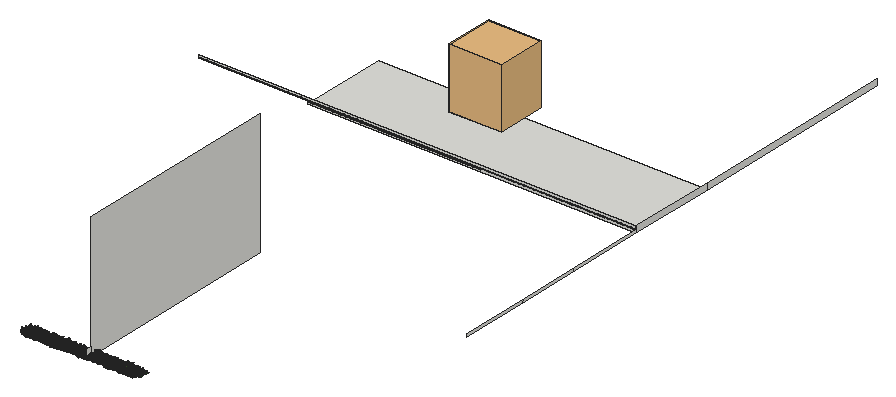
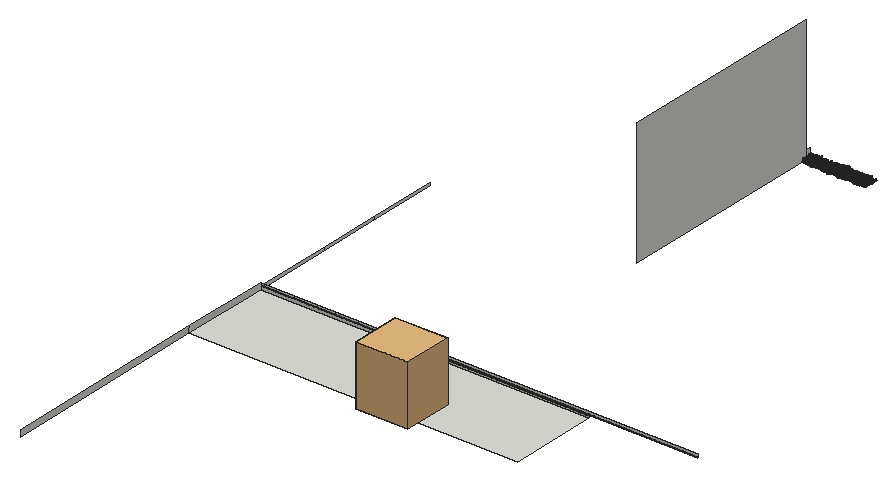
# SketchUp Ruby script. Lengths in inches.
U = 1.inch
M = Sketchup.active_model
def pt(a) = Geom::Point3d.new(a.map { |v| v * U })
def face(e, loops, mat)
  f = e.add_face(loops[0].map { |a| pt(a) })
  loops[1..].each { |l| e.add_face(l.map { |a| pt(a) }).erase! }
  f.material = f.back_material = mat if mat
  f
end
# faces: each face lists its corners as indices into pts; further lists are holes
def faces(e, pts, list, mat = nil) = list.each { |f| face(e, (f[0].is_a?(Array) ? f : [f]).map { |l| l.map { |i| pts[i] } }, mat) }
# xy, xz, yz: faces in a plane at the given z, y or x. An outline is a flat list of corners, or four numbers for a rectangle; further outlines are holes
def ring(l) = l.size == 4 ? [[l[0], l[1]], [l[2], l[1]], [l[2], l[3]], [l[0], l[3]]] : l.each_slice(2).to_a
def flat(e, list, mat, &to3) = list.each { |f| face(e, (f[0].is_a?(Array) ? f : [f]).map { |l| ring(l).map { |u, v| to3.(u, v) } }, mat) }
def xy(e, z, list, mat = nil) = flat(e, list, mat) { |x, y| [x, y, z] }
def xz(e, y, list, mat = nil) = flat(e, list, mat) { |x, z| [x, y, z] }
def yz(e, x, list, mat = nil) = flat(e, list, mat) { |y, z| [x, y, z] }
def lines(e, pts, list) = list.each { |a, b| e.add_line(pt(pts[a]), pt(pts[b])) }
# prism: a flat outline (further loops are holes) pulled along v
def prism(e, loops, v, mat = nil)
  f = face(e, loops, mat); d = Geom::Vector3d.new(v.map { |x| x * U })
  f.pushpull(f.normal.samedirection?(d) ? d.length : -d.length)
end
def box(e, o, s, mat = nil) = prism(e, [[o, [o[0] + s[0], o[1], o[2]], [o[0] + s[0], o[1] + s[1], o[2]], [o[0], o[1] + s[1], o[2]]]], [0, 0, s[2]], mat)
def at(x, y, z, deg = 0) = Geom::Transformation.translation(pt([x, y, z])) * Geom::Transformation.rotation(ORIGIN, Z_AXIS, deg.degrees)
def axes(o, x, y, z) = Geom::Transformation.new([*x, 0, *y, 0, *z, 0, *pt(o).to_a, 1])
def part(name) = M.definitions.add(name)
# library, detail: a bought-in or finely detailed component or shape, given as its bounding box
def library(name, o, s) = part(name).tap { |d| box(d.entities, o, s) }
def detail(e, o, s) = box(e.add_group.entities, o, s)
def put(e, d, t, mat = nil) = e.add_instance(d, t).tap { |i| i.material = mat if mat }
def group(e, t, mat = nil) = e.add_group.tap { |g| g.transformation = t; g.material = mat if mat }.entities
root = M.entities
M.materials.add("Material82").color = [68, 110, 58]
M.materials.add("Material83").color = [48, 90, 38]
M.materials.add("Material84").color = [68, 110, 48]
M.materials.add("Material85").color = [48, 90, 48]
M.materials.add("Material86").color = [58, 110, 58]
M.materials.add("Material87").color = [58, 90, 38]
M.materials.add("Material88").color = [68, 100, 58]
M.materials.add("Material89").color = [48, 100, 38]
c1 = part("grass00")
p = [[-0.6875,0.15,0],[-0.56,0.08,5.52],[-0.04,0.03,2.76],[0.48,-0.02,0],[0.35,-0.02,5.52],[-0.1,-0.14,5.52],
  [-0.12,0.65,8.37],[-0.42,0.65,8.37]]
faces(c1.entities,p,[[0,1,2,3],[3,2,4],[1,5,2],[5,4,2],[1,6,5],[4,5,6],[7,6,1]])
c2 = part("Group16\#1")
put(c2.entities,c1,axes([1.44,-0.61,-0.01],[0.05352,0.12609,0],[-0.10704,0.04543,0.07239],[0.06664,-0.02828,0.11628]),"Material85")
put(c2.entities,c1,axes([0.76,-0.15,-0.01],[0.04676,0.24062,0],[-0.23162,0.04501,0.06642],[0.0652,-0.01267,0.23595]),"Material82")
put(c2.entities,c1,axes([0.79,0.01,-0.01],[-0.00606,0.34651,0],[-0.34381,-0.00602,0.0432],[0.04319,0.00076,0.34386]))
put(c2.entities,c1,axes([1,0.23,-0.01],[-0.07192,0.31144,0],[-0.28722,-0.06632,0.1236],[0.12043,0.02781,0.29478]),"Material84")
put(c2.entities,c1,axes([1.66,0.77,-0.01],[-0.13828,0.29651,0],[-0.21551,-0.1005,0.22471],[0.20365,0.09498,0.23779]),"Material89")
put(c2.entities,c1,axes([0.6875,0.52,-0.01],[-0.18126,0.24051,0],[-0.22746,-0.17142,0.09788],[0.07817,0.05891,0.28481]),"Material84")
put(c2.entities,c1,axes([0.68,0.78,-0.01],[-0.215,0.18688,0],[-0.12385,-0.14248,0.21334],[0.13995,0.16101,0.18878]),"Material82")
put(c2.entities,c1,axes([0.56,1,-0.01],[-0.13756,0.07624,0],[-0.06159,-0.11112,0.0927],[0.04494,0.08108,0.12705]),"Material84")
put(c2.entities,c1,axes([0.2,0.64,-0.01],[-0.23729,0.07254,0],[-0.05711,-0.18681,0.153],[0.04473,0.14632,0.19535]),"Material89")
put(c2.entities,c1,axes([0.0625,0.72,-0.01],[-0.28874,0.02525,0],[-0.02179,-0.24916,0.14647],[0.01276,0.14591,0.25012]),"Material82")
put(c2.entities,c1,axes([-0.08,0.62,-0.01],[-0.34089,-0.04187,0],[0.03255,-0.26504,0.216],[-0.02633,0.21439,0.26703]),"Material89")
put(c2.entities,c1,axes([-0.34,0.98,-0.01],[-0.14314,-0.0493,0],[0.04397,-0.12769,0.06843],[-0.02228,0.0647,0.13505]),"Material89")
put(c2.entities,c1,axes([-0.87,1.45,-0.01],[-0.23488,-0.14114,0],[0.13761,-0.22901,0.06087],[-0.03135,0.05217,0.26717]))
put(c2.entities,c1,axes([-0.72,0.77,-0.01],[-0.14208,-0.13251,0],[0.07209,-0.0773,0.16301],[-0.11118,0.11922,0.1057]),"Material89")
put(c2.entities,c1,axes([-0.62,0.43,-0.01],[-0.14845,-0.21203,0],[0.18654,-0.13061,0.12304],[-0.10079,0.07057,0.22772]),"Material82")
put(c2.entities,c1,axes([-0.68,0.29,-0.01],[-0.13639,-0.32136,0],[0.31723,-0.13464,0.05579],[-0.05136,0.0218,0.34462]),"Material83")
put(c2.entities,c1,axes([-0.64,0.125,-0.01],[-0.0458,-0.23569,0],[0.22124,-0.043,0.08276],[-0.08124,0.01579,0.22538]),"Material86")
put(c2.entities,c1,axes([-1.6,-0.03,-0.01],[0.00576,-0.32897,0],[0.27526,0.00482,0.18018],[-0.18015,-0.00315,0.2753]),"Material84")
put(c2.entities,c1,axes([-1.36,-0.31,-0.01],[0.05718,-0.24765,0],[0.18172,0.04196,0.17267],[-0.16825,-0.03885,0.1865]),"Material89")
put(c2.entities,c1,axes([-1.54,-0.72,-0.01],[0.06537,-0.14017,0],[0.13555,0.06321,0.03939],[-0.0357,-0.01665,0.14956]))
put(c2.entities,c1,axes([-1.19,-0.9,-0.01],[0.09597,-0.12735,0],[0.11214,0.08451,0.07557],[-0.06035,-0.04548,0.14042]),"Material88")
put(c2.entities,c1,axes([-0.47,-0.54,-0.01],[0.11588,-0.10072,0],[0.0618,0.0711,0.12124],[-0.07953,-0.0915,0.0942]))
put(c2.entities,c1,axes([-0.47,-0.84,-0.01],[0.11927,-0.0661,0],[0.06603,0.11913,0.00646],[-0.00313,-0.00565,0.13621]),"Material84")
put(c2.entities,c1,axes([-0.38,-1.24,-0.01],[0.28037,-0.08571,0],[0.0618,0.20215,0.20315],[-0.05939,-0.19428,0.21139]),"Material88")
put(c2.entities,c1,axes([-0.06,-0.66,-0.01],[0.22719,-0.01987,0],[0.01247,0.14255,0.17758],[-0.01547,-0.17691,0.1431]),"Material87")
put(c2.entities,c1,axes([0.11,-0.89,-0.01],[0.14882,0.01828,0],[-0.01058,0.08611,0.12229],[0.01491,-0.12138,0.08676]),"Material85")
put(c2.entities,c1,axes([0.25,-0.72,-0.01],[0.20481,0.07053,0],[-0.06206,0.18022,0.10291],[0.03351,-0.0973,0.1906]),"Material85")
put(c2.entities,c1,axes([0.85,-1.42,-0.01],[0.16481,0.09904,0],[-0.09472,0.15762,0.05616],[0.02893,-0.04814,0.18389]),"Material84")
put(c2.entities,c1,axes([1.01,-1.09,-0.01],[0.21858,0.20385,0],[-0.17495,0.1876,0.15339],[0.10462,-0.11218,0.25652]),"Material89")
put(c2.entities,c1,axes([1.01,-0.71,-0.01],[0.08733,0.12473,0],[-0.06445,0.04512,0.13037],[0.1068,-0.07477,0.07867]),"Material85")
c3 = part("Group15\#1")
put(c3.entities,c2,at(0,0,0))
c4 = part("3darcstudiotree_grass00\#1")
put(c4.entities,c3,at(0,0,0))
c5 = library("Flora+17",[-57.52,158.6,-38.64],[66.99,62.88,77.28])
xy(root,-37.75,[[626.34,932.5,1048.3125,1046.93]])
xz(root,932.5,[[626.34,-37.75,1048.3125,-37.75,1048.3125,-34.17,848.625,-34.17,848.625,-34.6875,626.34,-34.6875],[626.34,-34.6875,848.625,-34.17],[626.34,-34.17,1048.3125,-33.75],[486.07,-33.75,1048.3125,-33.42],[486.07,-33.42,1048.3125,-32.8],
  [486.07,-32.8,1048.3125,-29.74]])
yz(root,782.78,[[381.72,-34.17,387.84,-22.8],[387.84,-34.17,659.09,126.75]])
yz(root,1048.3125,[[660.69,-37.75,750.06,-34.75],[750.06,-37.75,831.37,-34.75],[831.37,-37.75,932.5,-34.17],[932.5,-37.75,1046.93,-37.75,1046.93,-29.74,932.62,-29.74,932.62,-33.625,932.5,-33.625],[1046.93,-37.75,1318.18,-29.74],
  [932.5,-33.625,932.62,-29.74]])
put(root,c4,axes([730.45,381.9375,-34.17],[4.09331,0.01199,0],[-0.0289,1.53398,-0.04293],[-0.00148,0.07869,1.35522]))
put(root,c4,axes([778.3125,381.87,-34.17],[-3.29126,-0.79109,0],[1.80045,-1.16502,-0.03312],[0.11366,-0.07354,1.70984]))
put(root,c4,axes([741.45,381.79,-34.17],[1.86032,1.34861,0],[-2.96544,0.63621,-0.01685],[-0.11323,0.02429,1.93576]))
put(root,c4,axes([736.73,381.58,-34.17],[-4.56188,0.50767,0],[-1.2186,-1.7031,-0.00145],[-0.00214,-0.00299,1.8291]))
put(root,c4,axes([707.26,382.11,-34.17],[-1.58728,-1.19948,0],[3.58979,-0.73882,-0.00435],[0.01908,-0.00393,1.50222]))
put(root,c4,axes([720.02,382,-34.17],[-3.20908,-0.65771,0],[1.52004,-1.1535,-0.02241],[0.0705,-0.0535,1.68548]))
put(root,c4,axes([811.23,381.91,-34.17],[0.845,1.5364,0],[-3.22221,0.27563,-0.00976],[-0.06274,0.00537,1.62508]))
put(root,c4,axes([749.48,382.19,-34.17],[-3.10229,-1.16988,0],[2.93363,-1.20992,-0.00934],[0.03186,-0.01314,1.57129]))
put(root,c4,axes([835.72,382.97,-34.17],[3.21747,0.34612,0],[-1.00705,1.45598,-0.00322],[-0.00588,0.0085,1.99197]))
put(root,c4,axes([807.45,383.26,-34.17],[2.05313,-1.14667,0],[3.04328,0.84748,-0.00946],[0.04471,0.01245,1.61646]))
put(root,c4,axes([710.89,382.88,-34.17],[1.49785,1.29889,0],[-3.32043,0.59552,-0.00419],[-0.02419,0.00434,1.73548]))
put(root,c4,axes([828.28,383.19,-34.17],[-2.06721,-1.47479,0],[2.97534,-0.64864,-0.04183],[0.21369,-0.04658,1.48723]))
put(root,c4,axes([756.44,383.36,-34.17],[3.7963,-0.32727,0],[0.82791,1.49367,-0.02018],[0.02229,0.04022,1.50307]))
put(root,c4,axes([766.5,383.2,-34.17],[3.44974,0.13102,0],[-0.35474,1.45265,-0.03978],[-0.02715,0.11118,1.9745]))
put(root,c4,axes([814.17,383.25,-34.17],[3.55632,0.05998,0],[-0.17821,1.64336,-0.05798],[-0.01271,0.11725,1.60438]))
put(root,c4,axes([838.5,382.91,-34.17],[-3.26011,-0.21751,0],[0.57833,-1.34815,-0.02254],[0.02017,-0.04702,1.39425]))
put(root,c4,axes([773.79,383.16,-34.17],[-2.04014,-1.04561,0],[3.14641,-0.95481,-0.03027],[0.11908,-0.03613,1.47708]))
put(root,c4,axes([750.16,382.96,-34.17],[-4.12072,-0.27119,0],[0.6549,-1.54771,-0.03361],[0.02858,-0.06755,1.54092]))
put(root,c4,axes([707.83,383.13,-34.17],[-3.19208,-0.59663,0],[1.68588,-1.40285,-0.03887],[0.08271,-0.06882,1.46596]))
put(root,c4,axes([717.11,383.21,-34.17],[-3.36658,1.12781,0],[-2.16506,-1.00516,-0.00331],[-0.01262,-0.00586,1.47415]))
put(root,c4,axes([723.95,383.34,-34.17],[-3.68407,-0.02356,0],[0.06081,-1.47897,-0.00434],[0.00034,-0.00838,1.37632]))
put(root,c4,axes([795.54,384.11,-34.17],[3.71353,-0.51552,0],[1.56304,1.75115,-0.03514],[0.05159,0.0578,1.55988]))
put(root,c4,axes([747.36,383.45,-34.17],[0.6827,1.82438,0],[-3.27697,0.19072,-0.00575],[-0.03023,0.00176,1.31904]))
put(root,c4,axes([741.45,383.66,-34.17],[2.40726,1.00896,0],[-2.45133,0.90962,-0.04643],[-0.23456,0.08704,1.7498]))
put(root,c4,axes([734.375,384.03,-34.17],[0.00434,-1.45328,0],[3.77222,0.00175,-0.01884],[0.09694,0.00004,1.45492]))
put(root,c4,axes([817.26,384.18,-34.17],[1.06558,-1.7102,0],[3.88793,0.37676,-0.05295],[0.33853,0.03281,1.97565]))
put(root,c4,axes([763.28,383.8,-34.17],[-4.10821,-0.63147,0],[1.40621,-1.42285,-0.03755],[0.0732,-0.07407,1.55797]))
put(root,c4,axes([779.07,384.18,-34.17],[3.5779,0.22372,0],[-0.65952,1.64048,-0.02805],[-0.02776,0.06904,1.99488]))
put(root,c4,axes([790,384.14,-34.17],[-0.99859,-1.42329,0],[3.17499,-0.34645,-0.0133],[0.07574,-0.00827,1.45899]))
put(root,c4,axes([785.29,383.61,-34.17],[-2.82382,0.83563,0],[-2.68315,-1.4102,-0.02868],[-0.0714,-0.03753,1.39]))
put(root,c4,axes([824.1875,383.98,-34.17],[-4.01729,-0.17274,0],[0.40562,-1.46709,-0.05296],[0.03317,-0.11998,1.62079]))
put(root,c4,axes([729.49,383.9,-34.17],[-4.10797,-0.04724,0],[0.09871,-1.33508,-0.0193],[0.00442,-0.0598,1.99558]))
put(root,c4,axes([801.06,384.04,-34.17],[-1.96777,1.0795,0],[-3.29786,-0.93497,-0.0015],[-0.00541,-0.00153,1.35234]))
put(root,c4,axes([768.48,385.02,-34.17],[0.94515,-1.66762,0],[4.07339,0.35906,-0.0396],[0.18346,0.01617,1.48525]))
put(root,c4,axes([818.375,385.11,-34.17],[3.84561,-0.02617,0],[0.07345,1.67847,-0.0287],[0.00308,0.07036,1.98369]))
put(root,c4,axes([794.87,385.32,-34.17],[1.96372,-1.5045,0],[4.10696,0.83372,-0.06088],[0.26019,0.05282,1.6642]))
put(root,c4,axes([807.73,385.28,-34.17],[3.54187,-0.26159,0],[0.80325,1.69151,-0.05648],[0.04449,0.09368,1.39957]))
put(root,c4,axes([778,385.49,-34.17],[0.99321,-1.58581,0],[3.96504,0.38623,-0.04714],[0.20087,0.01957,1.34372]))
put(root,c4,axes([763.58,385.62,-34.17],[-0.45128,-1.33361,0],[4.22591,-0.22241,-0.03174],[0.17504,-0.00921,1.77768]))
put(root,c4,axes([745.49,385.82,-34.17],[3.22644,-0.51746,0],[1.32565,1.28555,-0.02601],[0.05462,0.05297,1.4702]))
put(root,c4,axes([725.2,385.76,-34.17],[3.6798,1.00569,0],[-2.52504,1.43694,-0.01195],[-0.02817,0.01603,1.37528]))
put(root,c4,axes([789.81,385.57,-34.17],[1.82247,1.66574,0],[-4.14446,0.70523,-0.02206],[-0.09849,0.01676,1.64521]))
put(root,c4,axes([749.67,385.65,-34.17],[-2.84959,-0.68183,0],[2.166,-1.40791,-0.04577],[0.14869,-0.09665,1.96036]))
put(root,c4,axes([771.69,385.93,-34.17],[4.19345,0.64908,0],[-1.43857,1.4455,-0.00074],[-0.00143,0.00144,1.56313]))
put(root,c4,axes([813.67,385.29,-34.17],[-3.99369,0.93834,0],[-2.11578,-1.40055,-0.00882],[-0.02078,-0.01375,1.42641]))
put(root,c4,axes([827.56,385.48,-34.17],[-3.34892,0.63546,0],[-1.79553,-1.4717,-0.05656],[-0.12201,-0.10001,1.54444]))
put(root,c4,axes([757.6,386.15,-34.17],[2.39093,-1.03283,0],[3.02488,1.08907,-0.05494],[0.24262,0.08735,1.83588]))
put(root,c4,axes([823.76,385.55,-34.17],[-2.29973,1.37871,0],[-3.78776,-0.98265,-0.04701],[-0.18775,-0.04871,1.62457]))
put(root,c4,axes([717.05,385.77,-34.17],[0.30119,1.56993,0],[-3.74927,0.11187,-0.04286],[-0.21599,0.00644,1.42447]))
put(root,c4,axes([837.94,386.3,-34.17],[4.21864,0.55626,0],[-1.1609,1.36932,-0.01696],[-0.03551,0.04188,1.81122]))
put(root,c4,axes([734.35,385.875,-34.17],[-3.66261,0.69653,0],[-1.57298,-1.28643,-0.02015],[-0.06083,-0.04975,1.88684]))
put(root,c4,axes([801.61,385.9,-34.17],[-0.80631,1.56039,0],[-4.1673,-0.33492,-0.00834],[-0.04436,-0.00356,1.72954]))
put(root,c4,axes([705.41,386.3,-34.17],[-0.23965,1.40351,0],[-3.9598,-0.10516,-0.04305],[-0.25813,-0.00685,1.78778]))
put(root,c4,axes([731.27,386.33,-34.17],[-0.04316,1.58062,0],[-4.72981,-0.02009,-0.05791],[-0.26281,-0.00112,1.60897]))
put(root,c4,axes([833.79,386.28,-34.17],[-3.37719,0.09425,0],[-0.3007,-1.67585,-0.01026],[-0.00386,-0.0215,1.70108]))
put(root,c4,axes([738.7,386.49,-34.17],[0.64791,1.78613,0],[-4.32576,0.24405,-0.02596],[-0.10407,0.00587,1.32635]))
put(root,c4,axes([712.38,386.58,-34.17],[-3.52632,-0.01876,0],[0.05142,-1.50323,-0.03579],[0.00272,-0.07942,1.60809]))
put(root,c4,axes([786.09,386.45,-34.17],[-1.94441,1.40342,0],[-3.94861,-0.85085,-0.04785],[-0.22127,-0.04768,1.77706]))
put(root,c4,axes([729.53,387.22,-34.17],[0.58086,-1.47611,0],[3.37891,0.2068,-0.00401],[0.02817,0.00172,1.82024]))
put(root,c4,axes([834.7,387.4375,-34.17],[3.52188,-1.04915,0],[2.07703,1.0844,-0.01203],[0.05383,0.0281,1.91781]))
put(root,c4,axes([758.35,387.51,-34.17],[-0.2827,-1.72948,0],[4.63241,-0.11777,-0.03565],[0.15653,-0.00398,1.53082]))
put(root,c4,axes([725.43,387.43,-34.17],[-3.67064,-0.9709,0],[1.88491,-1.10833,-0.03319],[0.11926,-0.07012,1.63594]))
put(root,c4,axes([717.875,387.83,-34.17],[3.50639,-1.07574,0],[2.8139,1.42651,-0.05588],[0.16686,0.08459,1.67045]))
put(root,c4,axes([812.48,387.78,-34.17],[1.01558,-1.39222,0],[4.1939,0.47581,-0.0144],[0.07646,0.00867,1.80693]))
put(root,c4,axes([773.38,387.48,-34.17],[3.41924,1.14131,0],[-2.67356,1.24575,-0.04954],[-0.1842,0.08583,1.78537]))
put(root,c4,axes([799.93,387.26,-34.17],[0.28845,1.63387,0],[-3.6901,0.10132,-0.01352],[-0.07291,0.002,1.49862]))
put(root,c4,axes([711.25,387.49,-34.17],[2.65644,1.45338,0],[-3.09672,0.88031,-0.01552],[-0.06337,0.01801,1.43977]))
put(root,c4,axes([782.6875,387.98,-34.17],[1.87129,-1.65871,0],[3.35394,0.58849,-0.03607],[0.16948,0.02974,1.41495]))
put(root,c4,axes([838.375,387.96,-34.17],[3.01548,-1.43579,0],[2.66285,0.86981,-0.04892],[0.23141,0.07559,1.59182]))
put(root,c4,axes([745.71,387.43,-34.17],[-3.80321,-0.44648,0],[1.10938,-1.46975,-0.0137],[0.0187,-0.02478,1.39479]))
put(root,c4,axes([829.69,387.32,-34.17],[-3.21998,0.77713,0],[-2.13854,-1.37813,-0.04749],[-0.1058,-0.06818,1.3106]))
put(root,c4,axes([822.12,388.125,-34.17],[4.18213,-0.23196,0],[0.63555,1.78214,-0.01318],[0.01066,0.02989,1.98636]))
put(root,c4,axes([763.71,388.09,-34.17],[-2.48368,-1.57939,0],[3.38438,-0.82775,-0.05324],[0.27998,-0.06848,1.84703]))
put(root,c4,axes([794.69,388.25,-34.17],[4.18444,0.27637,0],[-0.72897,1.71663,-0.00046],[-0.00033,0.00077,1.40239]))
put(root,c4,axes([807.18,388.3,-34.17],[3.48402,0.19943,0],[-0.6366,1.72969,-0.0224],[-0.01372,0.03729,1.41716]))
put(root,c4,axes([791.91,388.375,-34.17],[2.76674,0.9412,0],[-2.67302,1.22208,-0.02494],[-0.08686,0.03971,1.63549]))
put(root,c4,axes([739.22,388.16,-34.17],[2.43664,1.45627,0],[-2.82206,0.73439,-0.04277],[-0.22349,0.05816,1.58679]))
put(root,c4,axes([818.81,388.69,-34.17],[1.32588,-1.61709,0],[3.49004,0.44505,-0.02554],[0.12415,0.01583,1.40467]))
put(root,c4,axes([779.86,388.49,-34.17],[3.90165,0.71674,0],[-1.5443,1.30747,-0.0112],[-0.02712,0.02296,1.5714]))
put(root,c4,axes([766.36,388.28,-34.17],[-2.56197,0.85481,0],[-2.91428,-1.35846,-0.04396],[-0.15305,-0.07134,1.82298]))
put(root,c4,axes([735.62,388.47,-34.17],[-0.0946,1.80399,0],[-4.6355,-0.03781,-0.04199],[-0.20347,-0.00166,1.68448]))
put(root,c4,axes([752.28,388.59,-34.17],[-3.95195,-0.11479,0],[0.31612,-1.69258,-0.00991],[0.00383,-0.02049,1.69565]))
put(root,c4,axes([791.42,389.54,-34.17],[2.92757,-1.05075,0],[2.58194,1.11883,-0.00947],[0.03015,0.01306,1.36019]))
put(root,c4,axes([734.5,389.5625,-34.17],[4.14299,-0.56741,0],[1.47163,1.6712,-0.03586],[0.0631,0.07166,1.80381]))
put(root,c4,axes([813.64,389.64,-34.17],[2.43403,-1.47369,0],[3.95187,1.01516,-0.04483],[0.17665,0.04538,1.66248]))
put(root,c4,axes([741.56,389.7,-34.17],[2.20641,-0.98098,0],[3.35125,1.17232,-0.037],[0.12603,0.04409,1.52862]))
put(root,c4,axes([800.07,389.625,-34.17],[-0.61871,-1.33799,0],[4.52735,-0.32561,-0.01194],[0.05418,-0.0039,1.59034]))
put(root,c4,axes([766.42,389.36,-34.17],[-3.07207,1.32257,0],[-2.98229,-1.07739,-0.02313],[-0.10886,-0.03933,1.93523]))
put(root,c4,axes([824.82,389.9,-34.17],[-2.58829,-1.32174,0],[3.13096,-0.95358,-0.00917],[0.03927,-0.01196,1.60374]))
put(root,c4,axes([758.55,389.68,-34.17],[1.17272,1.70605,0],[-3.75992,0.40197,-0.02312],[-0.1149,0.01228,1.50331]))
put(root,c4,axes([836.33,389.68,-34.17],[0.77928,1.7442,0],[-4.29167,0.29822,-0.04576],[-0.22745,0.0158,1.64855]))
put(root,c4,axes([727.98,390.06,-34.17],[-3.05504,-0.78096,0],[2.06441,-1.25601,-0.04254],[0.14556,-0.08856,1.78955]))
put(root,c4,axes([806.71,389.87,-34.17],[-0.96871,1.48497,0],[-4.54289,-0.46091,-0.03008],[-0.14643,-0.01486,1.76703]))
put(root,c4,axes([705.875,389.98,-34.17],[0.67536,1.71011,0],[-3.33591,0.2049,-0.00889],[-0.04851,0.00298,1.39664]))
put(root,c4,axes([777.59,390.38,-34.17],[2.90547,0.96842,0],[-2.50521,1.16898,-0.00305],[-0.01073,0.00501,1.58836]))
put(root,c4,axes([751.86,390.13,-34.17],[-4.49885,0.1512,0],[-0.3136,-1.45126,-0.04489],[-0.02566,-0.11876,1.86365]))
put(root,c4,axes([775.48,390.39,-34.17],[-2.30012,-1.16982,0],[2.63485,-0.80575,-0.0081],[0.04804,-0.01469,1.87526]))
put(root,c4,axes([795.52,390.18,-34.17],[-3.42471,-0.0278,0],[0.09598,-1.83904,-0.05231],[0.00587,-0.11256,1.90792]))
put(root,c4,axes([784.88,390.48,-34.17],[-1.92512,-1.14787,0],[3.14134,-0.81939,-0.00554],[0.02611,-0.00681,1.59445]))
put(root,c4,axes([718.41,390.12,-34.17],[-1.98309,1.36521,0],[-3.29696,-0.74485,-0.00674],[-0.03007,-0.00679,1.46389]))
put(root,c4,axes([827.23,390.5,-34.17],[2.80131,1.49669,0],[-2.81369,0.81906,-0.03251],[-0.16371,0.04766,1.64081]))
put(root,c4,axes([761.27,390.83,-34.17],[3.47876,0.69717,0],[-2.07434,1.60981,-0.02666],[-0.05222,0.04053,1.48409]))
put(root,c4,axes([724.33,390.43,-34.17],[-2.752,0.72492,0],[-2.08218,-1.22939,-0.04884],[-0.13401,-0.07912,1.38796]))
put(root,c4,axes([714.3,390.3,-34.17],[-2.99935,1.42497,0],[-3.08029,-1.00838,-0.00469],[-0.01919,-0.00628,1.59556]))
put(root,c4,axes([745.25,390.95,-34.17],[-4.04158,-0.94067,0],[1.75814,-1.17484,-0.01139],[0.03404,-0.02275,1.52439]))
put(root,c4,axes([818.09,390.95,-34.17],[-2.36734,0.93793,0],[-2.35302,-0.92369,-0.04592],[-0.18701,-0.07341,1.42994]))
put(root,c4,axes([777.11,391.58,-34.17],[3.51961,1.01739,0],[-2.56437,1.37974,-0.04132],[-0.14142,0.07609,1.88254]))
put(root,c4,axes([719.25,391.75,-34.17],[-0.91614,-1.55858,0],[4.47177,-0.40881,-0.01344],[0.0544,-0.00497,1.42931]))
put(root,c4,axes([749.64,391.89,-34.17],[3.44355,0.26807,0],[-0.70938,1.41724,-0.02055],[-0.0272,0.05435,1.87683]))
put(root,c4,axes([746.7,392.14,-34.17],[4.25801,-0.4781,0],[1.08249,1.49942,-0.0361],[0.05003,0.0693,1.4995]))
put(root,c4,axes([802.02,391.64,-34.17],[-4.54557,-0.49368,0],[1.16722,-1.67149,-0.00177],[0.00248,-0.00355,1.73275]))
put(root,c4,axes([741.1,391.57,-34.17],[-3.5428,1.01388,0],[-2.21614,-1.2044,-0.01293],[-0.05166,-0.02807,1.92389]))
put(root,c4,axes([722.65,392.21,-34.17],[3.58378,0.39823,0],[-1.22974,1.72119,-0.04858],[-0.06101,0.08539,1.57379]))
put(root,c4,axes([764.43,391.72,-34.17],[-3.51929,1.02852,0],[-2.47816,-1.3188,-0.03727],[-0.13373,-0.07117,1.88005]))
put(root,c4,axes([817.71,392.18,-34.17],[2.58784,1.12355,0],[-2.76399,0.99014,-0.01914],[-0.07187,0.02574,1.41957]))
put(root,c4,axes([706.66,392.6,-34.17],[2.58879,-1.26718,0],[2.80569,0.89147,-0.02709],[0.14156,0.04498,1.8123]))
put(root,c4,axes([832.6875,392.74,-34.17],[3.2252,-1.24507,0],[3.05222,1.22967,-0.00616],[0.02183,0.0088,1.65812]))
put(root,c4,axes([791.12,392,-34.17],[-3.2702,-0.26148,0],[0.88726,-1.72581,-0.02938],[0.02304,-0.04482,1.3208]))
put(root,c4,axes([729.27,392.63,-34.17],[0.31357,-1.68647,0],[3.44554,0.09964,-0.00239],[0.01314,0.00038,1.42634]))
put(root,c4,axes([785.6,392.63,-34.17],[3.46613,-0.34597,0],[1.04996,1.63602,-0.03471],[0.05136,0.08002,1.93398]))
put(root,c4,axes([756.51,392.28,-34.17],[-3.51186,-0.721,0],[1.80955,-1.37083,-0.02288],[0.05511,-0.04175,1.53217]))
put(root,c4,axes([839.03,392.1,-34.17],[-1.83571,1.27258,0],[-3.25848,-0.73105,-0.04597],[-0.18825,-0.04223,1.32398]))
put(root,c4,axes([824.75,392.78,-34.17],[3.30404,-0.44467,0],[1.11823,1.29225,-0.02189],[0.05068,0.05857,1.86062]))
put(root,c4,axes([810.33,392.7,-34.17],[3.79709,-0.21086,0],[0.51761,1.44966,-0.04526],[0.04066,0.11387,1.7925]))
put(root,c4,axes([732.67,392.78,-34.17],[4.65922,-0.05932,0],[0.11762,1.43686,-0.01793],[0.0038,0.04639,1.79317]))
put(root,c4,axes([768.91,392.66,-34.17],[-2.71598,-1.39793,0],[3.51357,-1.0617,-0.04805],[0.18587,-0.05616,1.61679]))
put(root,c4,axes([805.43,392.33,-34.17],[-1.13728,1.56272,0],[-3.25789,-0.36875,-0.04255],[-0.28342,-0.03208,1.76068]))
put(root,c4,axes([794.21,393.07,-34.17],[3.34396,-0.78628,0],[2.01461,1.33256,-0.01626],[0.05098,0.03372,1.80561]))
put(root,c4,axes([827.74,392.48,-34.17],[-3.32221,0.63503,0],[-1.46009,-1.18802,-0.04774],[-0.13797,-0.11226,1.66266]))
put(root,c4,axes([774.99,392.63,-34.17],[-4.26955,0.05297,0],[-0.11438,-1.43394,-0.03177],[-0.00727,-0.09116,1.98473]))
put(root,c4,axes([712.03,393.07,-34.17],[-3.0378,0.91986,0],[-2.50548,-1.28689,-0.05552],[-0.17911,-0.092,1.63365]))
put(root,c4,axes([712.95,393.82,-34.17],[2.17543,-1.37172,0],[2.92508,0.72149,-0.0272],[0.16226,0.04002,1.81972]))
put(root,c4,axes([789.92,393.8,-34.17],[1.37568,-1.20584,0],[3.91752,0.6951,-0.04402],[0.22671,0.04023,1.81837]))
put(root,c4,axes([812.15,393.71,-34.17],[3.59871,0.46514,0],[-1.32691,1.59666,-0.04711],[-0.07156,0.0861,1.55738]))
put(root,c4,axes([799.91,393.91,-34.17],[-2.0544,-1.27697,0],[2.98947,-0.74801,-0.00968],[0.05342,-0.01337,1.73508]))
put(root,c4,axes([735.42,393.93,-34.17],[-1.59587,-1.14266,0],[4.12201,-0.89537,-0.06742],[0.26463,-0.05748,1.58058]))
put(root,c4,axes([838.85,394.33,-34.17],[3.62221,-0.68496,0],[1.51778,1.24833,-0.03326],[0.08982,0.07387,1.64345]))
put(root,c4,axes([830.09,393.89,-34.17],[-0.69326,1.7064,0],[-4.31448,-0.27262,-0.01053],[-0.04979,-0.00315,1.56894]))
put(root,c4,axes([825.39,394.22,-34.17],[2.26243,1.54744,0],[-3.43917,0.78203,-0.02249],[-0.10645,0.02421,1.62577]))
put(root,c4,axes([750.13,394.22,-34.17],[0.25287,1.52902,0],[-3.62555,0.09325,-0.03468],[-0.21891,0.00563,1.72254]))
put(root,c5,at(807.58,846.28,4.4375))
